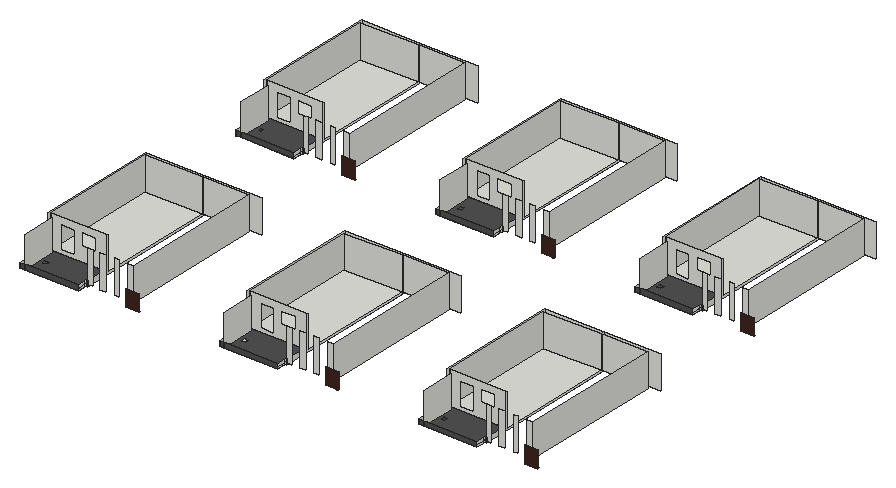
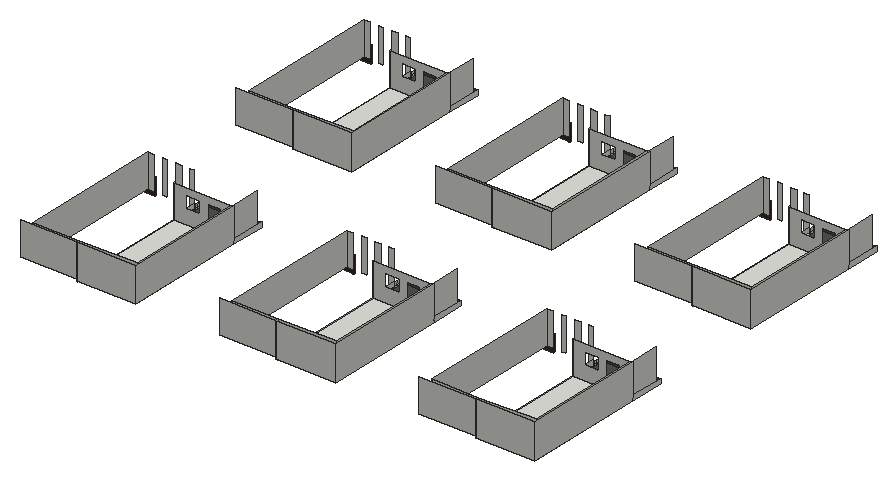
# SketchUp Ruby script. Lengths in inches.
U = 1.inch
M = Sketchup.active_model
def pt(a) = Geom::Point3d.new(a.map { |v| v * U })
def face(e, loops, mat)
  f = e.add_face(loops[0].map { |a| pt(a) })
  loops[1..].each { |l| e.add_face(l.map { |a| pt(a) }).erase! }
  f.material = f.back_material = mat if mat
  f
end
# faces: each face lists its corners as indices into pts; further lists are holes
def faces(e, pts, list, mat = nil) = list.each { |f| face(e, (f[0].is_a?(Array) ? f : [f]).map { |l| l.map { |i| pts[i] } }, mat) }
# xy, xz, yz: faces in a plane at the given z, y or x. An outline is a flat list of corners, or four numbers for a rectangle; further outlines are holes
def ring(l) = l.size == 4 ? [[l[0], l[1]], [l[2], l[1]], [l[2], l[3]], [l[0], l[3]]] : l.each_slice(2).to_a
def flat(e, list, mat, &to3) = list.each { |f| face(e, (f[0].is_a?(Array) ? f : [f]).map { |l| ring(l).map { |u, v| to3.(u, v) } }, mat) }
def xy(e, z, list, mat = nil) = flat(e, list, mat) { |x, y| [x, y, z] }
def xz(e, y, list, mat = nil) = flat(e, list, mat) { |x, z| [x, y, z] }
def yz(e, x, list, mat = nil) = flat(e, list, mat) { |y, z| [x, y, z] }
def lines(e, pts, list) = list.each { |a, b| e.add_line(pt(pts[a]), pt(pts[b])) }
# prism: a flat outline (further loops are holes) pulled along v
def prism(e, loops, v, mat = nil)
  f = face(e, loops, mat); d = Geom::Vector3d.new(v.map { |x| x * U })
  f.pushpull(f.normal.samedirection?(d) ? d.length : -d.length)
end
def box(e, o, s, mat = nil) = prism(e, [[o, [o[0] + s[0], o[1], o[2]], [o[0] + s[0], o[1] + s[1], o[2]], [o[0], o[1] + s[1], o[2]]]], [0, 0, s[2]], mat)
def at(x, y, z, deg = 0) = Geom::Transformation.translation(pt([x, y, z])) * Geom::Transformation.rotation(ORIGIN, Z_AXIS, deg.degrees)
def axes(o, x, y, z) = Geom::Transformation.new([*x, 0, *y, 0, *z, 0, *pt(o).to_a, 1])
def part(name) = M.definitions.add(name)
# library, detail: a bought-in or finely detailed component or shape, given as its bounding box
def library(name, o, s) = part(name).tap { |d| box(d.entities, o, s) }
def detail(e, o, s) = box(e.add_group.entities, o, s)
def put(e, d, t, mat = nil) = e.add_instance(d, t).tap { |i| i.material = mat if mat }
def group(e, t, mat = nil) = e.add_group.tap { |g| g.transformation = t; g.material = mat if mat }.entities
root = M.entities
M.materials.add("[0043_SaddleBrown]").color = [63, 38, 31]
M.materials.add("[0135_DarkGray]").color = [81, 81, 81]
xy(root,114.29,[[500.42,438.72,500.42,441.04,547.05,441.04,547.05,438.73],[1224.86,438.72,1224.86,441.04,1271.49,441.04,1271.49,438.73],[1949.3,438.72,1949.3,441.04,1995.93,441.04,1995.93,438.73],[500.42,1419.07,500.42,1421.39,547.05,1421.39,547.05,1419.08],[1224.86,1419.07,1224.86,1421.39,1271.49,1421.39,1271.49,1419.08],
  [1949.3,1419.07,1949.3,1421.39,1995.93,1421.39,1995.93,1419.08]])
xy(root,126.125,[[348.1875,447.84,353.97,980.35],[1072.625,447.84,1078.41,980.35],[1797.0625,447.84,1802.84,980.35],[891.39,475.13,905.02,487.19],[891.39,567.38,905.02,579.44],
  [891.39,682.44,905.02,694.5],[891.39,858.25,905.02,870.31],[348.1875,1428.19,353.97,1960.7],[1072.625,1428.19,1078.41,1960.7],[1797.0625,1428.19,1802.84,1960.7]])
xy(root,126.125,[[137.5,412.04,153.26,535.375],[[153.26,412.04,348.1875,412.04,348.1875,971.23,137.5,971.23,137.5,535.375,153.26,535.375],[166.95,858.25,180.58,870.31],[166.95,682.44,180.58,694.5],[166.95,567.38,180.58,579.44],[166.95,475.13,180.58,487.19]],[861.9375,412.04,877.69,535.375],[877.69,412.04,877.69,535.375,861.9375,535.375,861.9375,971.23,1072.625,971.23,1072.625,412.04],[1586.375,412.04,1602.13,535.375],
  [[1602.13,412.04,1797.0625,412.04,1797.0625,971.23,1586.375,971.23,1586.375,535.375,1602.13,535.375],[1615.83,858.25,1629.45,870.31],[1615.83,682.44,1629.45,694.5],[1615.83,567.38,1629.45,579.44],[1615.83,475.13,1629.45,487.19]],[166.95,475.13,180.58,487.19],[1615.83,475.13,1629.45,487.19],[166.95,567.38,180.58,579.44],[1615.83,567.38,1629.45,579.44],
  [166.95,682.44,180.58,694.5],[1615.83,682.44,1629.45,694.5],[166.95,858.25,180.58,870.31],[1615.83,858.25,1629.45,870.31],[137.5,1392.39,153.26,1515.73],
  [[153.26,1392.39,348.1875,1392.39,348.1875,1951.58,137.5,1951.58,137.5,1515.73,153.26,1515.73],[166.95,1838.6,180.58,1850.66],[166.95,1662.79,180.58,1674.85],[166.95,1547.73,180.58,1559.79],[166.95,1455.48,180.58,1467.54]],[861.9375,1392.39,877.69,1515.73],[[877.69,1392.39,877.69,1515.73,861.9375,1515.73,861.9375,1951.58,1072.625,1951.58,1072.625,1392.39],[891.39,1455.48,905.02,1467.54],[891.39,1547.73,905.02,1559.79],[891.39,1662.79,905.02,1674.85],[891.39,1838.6,905.02,1850.66]],[1586.375,1392.39,1602.13,1515.73],[[1602.13,1392.39,1797.0625,1392.39,1797.0625,1951.58,1586.375,1951.58,1586.375,1515.73,1602.13,1515.73],[1615.83,1838.6,1629.45,1850.66],[1615.83,1662.79,1629.45,1674.85],[1615.83,1547.73,1629.45,1559.79],[1615.83,1455.48,1629.45,1467.54]],
  [166.95,1455.48,180.58,1467.54],[891.39,1455.48,905.02,1467.54],[1615.83,1455.48,1629.45,1467.54],[166.95,1547.73,180.58,1559.79],[891.39,1547.73,905.02,1559.79],
  [1615.83,1547.73,1629.45,1559.79],[166.95,1662.79,180.58,1674.85],[891.39,1662.79,905.02,1674.85],[1615.83,1662.79,1629.45,1674.85],[166.95,1838.6,180.58,1850.66],
  [891.39,1838.6,905.02,1850.66],[1615.83,1838.6,1629.45,1850.66]],"[0135_DarkGray]")
xy(root,132.25,[[144.84,540.48,353.97,540.48,353.97,971.23,144.84,965.96],[869.28,540.48,1078.41,540.48,1078.41,971.23,869.28,965.96],[1593.72,540.48,1802.84,540.48,1802.84,971.23,1593.72,965.96],[144.84,1520.83,353.97,1520.83,353.97,1951.58,144.84,1946.3125],[869.28,1520.83,1078.41,1520.83,1078.41,1951.58,869.28,1946.3125],
  [1593.72,1520.83,1802.84,1520.83,1802.84,1951.58,1593.72,1946.3125]])
xz(root,412.04,[[137.5,126.125,153.26,143.875],[153.26,126.125,348.1875,143.875],[861.9375,126.125,877.69,143.875],[877.69,126.125,1072.625,143.875],[1586.375,126.125,1602.13,143.875],
  [1602.13,126.125,1797.0625,143.875]],"[0135_DarkGray]")
xz(root,447.84,[[348.1875,126.125,353.97,132.25],[1072.625,126.125,1078.41,132.25],[1797.0625,126.125,1802.84,132.25],[348.1875,132.25,353.97,143.875],[353.97,132.25,370.54,252.25],
  [399.16,132.25,419.76,252.25],[451.01,132.25,467.3,252.25],[500.42,132.25,521.63,252.25],[1072.625,132.25,1078.41,143.875],[1078.41,132.25,1094.98,252.25],
  [1123.6,132.25,1144.2,252.25],[1175.45,132.25,1191.74,252.25],[1224.86,132.25,1246.07,252.25],[1797.0625,132.25,1802.84,143.875],[1802.84,132.25,1819.41,252.25],
  [1848.04,132.25,1868.64,252.25],[1899.89,132.25,1916.17,252.25],[1949.3,132.25,1970.51,252.25]])
xz(root,535.375,[[137.5,126.125,153.26,143.875],[861.9375,126.125,877.69,143.875],[1586.375,126.125,1602.13,143.875]])
xz(root,540.48,[[[144.84,132.25,353.97,252.25],[183.3,143.875,231.3,227.875],[258.09,183.6875,309.84,227.875]],[[869.28,132.25,1078.41,252.25],[907.74,143.875,955.74,227.875],[982.53,183.6875,1034.28,227.875]],[[1593.72,132.25,1802.84,252.25],[1632.17,143.875,1680.17,227.875],[1706.96,183.6875,1758.71,227.875]]])
xz(root,971.23,[[353.97,132.25,521.63,252.25],[1078.41,132.25,1246.07,252.25],[1802.84,132.25,1970.51,252.25]])
xz(root,980.35,[[137.5,126.125,353.97,252.25],[861.9375,126.125,1078.41,252.25],[1586.375,126.125,1802.84,252.25],[353.97,132.25,558.625,252.25],[1078.41,132.25,1283.0625,252.25],
  [1802.84,132.25,2007.5,252.25]])
xz(root,1392.39,[[137.5,126.125,153.26,143.875],[153.26,126.125,348.1875,143.875],[861.9375,126.125,877.69,143.875],[877.69,126.125,1072.625,143.875],[1586.375,126.125,1602.13,143.875],
  [1602.13,126.125,1797.0625,143.875]],"[0135_DarkGray]")
xz(root,1428.19,[[348.1875,126.125,353.97,132.25],[1072.625,126.125,1078.41,132.25],[1797.0625,126.125,1802.84,132.25],[348.1875,132.25,353.97,143.875],[353.97,132.25,370.54,252.25],
  [399.16,132.25,419.76,252.25],[451.01,132.25,467.3,252.25],[500.42,132.25,521.63,252.25],[1072.625,132.25,1078.41,143.875],[1078.41,132.25,1094.98,252.25],
  [1123.6,132.25,1144.2,252.25],[1175.45,132.25,1191.74,252.25],[1224.86,132.25,1246.07,252.25],[1797.0625,132.25,1802.84,143.875],[1802.84,132.25,1819.41,252.25],
  [1848.04,132.25,1868.64,252.25],[1899.89,132.25,1916.17,252.25],[1949.3,132.25,1970.51,252.25]])
xz(root,1515.73,[[137.5,126.125,153.26,143.875],[861.9375,126.125,877.69,143.875],[1586.375,126.125,1602.13,143.875]])
xz(root,1520.83,[[[144.84,132.25,353.97,252.25],[183.3,143.875,231.3,227.875],[258.09,183.6875,309.84,227.875]],[[869.28,132.25,1078.41,252.25],[907.74,143.875,955.74,227.875],[982.53,183.6875,1034.28,227.875]],[[1593.72,132.25,1802.84,252.25],[1632.17,143.875,1680.17,227.875],[1706.96,183.6875,1758.71,227.875]]])
xz(root,1951.58,[[353.97,132.25,521.63,252.25],[1078.41,132.25,1246.07,252.25],[1802.84,132.25,1970.51,252.25]])
xz(root,1960.7,[[137.5,126.125,353.97,252.25],[861.9375,126.125,1078.41,252.25],[1586.375,126.125,1802.84,252.25],[353.97,132.25,558.625,252.25],[1078.41,132.25,1283.0625,252.25],
  [1802.84,132.25,2007.5,252.25]])
yz(root,137.5,[[412.04,126.125,535.375,143.875],[535.375,126.125,980.35,252.25],[1392.39,126.125,1515.73,143.875],[1515.73,126.125,1960.7,252.25]])
yz(root,144.84,[[540.48,132.25,965.96,252.25],[1520.83,132.25,1946.3125,252.25]])
yz(root,153.26,[[412.04,126.125,535.375,240.625],[1392.39,126.125,1515.73,240.625]])
yz(root,348.1875,[[412.04,126.125,438.72,132.25],[438.72,126.125,447.84,132.25],[1392.39,126.125,1419.07,132.25],[1419.07,126.125,1428.19,132.25],[412.04,132.25,438.72,143.875],
  [438.72,132.25,447.84,143.875],[1392.39,132.25,1419.07,143.875],[1419.07,132.25,1428.19,143.875]])
yz(root,353.97,[[447.84,126.125,971.23,126.125,971.23,132.25,540.48,132.25,540.48,252.25,535.375,252.25,535.375,143.875,447.84,143.875],[971.23,126.125,980.35,132.25],[1428.19,126.125,1951.58,126.125,1951.58,132.25,1520.83,132.25,1520.83,252.25,1515.73,252.25,1515.73,143.875,1428.19,143.875],[1951.58,126.125,1960.7,132.25],[971.23,132.25,980.35,252.25],
  [1951.58,132.25,1960.7,252.25]])
yz(root,521.63,[[447.84,132.25,971.23,252.25],[1428.19,132.25,1951.58,252.25]])
yz(root,861.9375,[[412.04,126.125,535.375,143.875],[535.375,126.125,980.35,252.25],[1392.39,126.125,1515.73,143.875],[1515.73,126.125,1960.7,252.25]])
yz(root,869.28,[[540.48,132.25,965.96,252.25],[1520.83,132.25,1946.3125,252.25]])
yz(root,877.69,[[412.04,126.125,535.375,240.625],[1392.39,126.125,1515.73,240.625]])
yz(root,1072.625,[[412.04,126.125,438.72,132.25],[438.72,126.125,447.84,132.25],[1392.39,126.125,1419.07,132.25],[1419.07,126.125,1428.19,132.25],[412.04,132.25,438.72,143.875],
  [438.72,132.25,447.84,143.875],[1392.39,132.25,1419.07,143.875],[1419.07,132.25,1428.19,143.875]])
yz(root,1078.41,[[447.84,126.125,971.23,126.125,971.23,132.25,540.48,132.25,540.48,252.25,535.375,252.25,535.375,143.875,447.84,143.875],[971.23,126.125,980.35,132.25],[1428.19,126.125,1951.58,126.125,1951.58,132.25,1520.83,132.25,1520.83,252.25,1515.73,252.25,1515.73,143.875,1428.19,143.875],[1951.58,126.125,1960.7,132.25],[971.23,132.25,980.35,252.25],
  [1951.58,132.25,1960.7,252.25]])
yz(root,1246.07,[[447.84,132.25,971.23,252.25],[1428.19,132.25,1951.58,252.25]])
yz(root,1586.375,[[412.04,126.125,535.375,143.875],[535.375,126.125,980.35,252.25],[1392.39,126.125,1515.73,143.875],[1515.73,126.125,1960.7,252.25]])
yz(root,1593.72,[[540.48,132.25,965.96,252.25],[1520.83,132.25,1946.3125,252.25]])
yz(root,1602.13,[[412.04,126.125,535.375,240.625],[1392.39,126.125,1515.73,240.625]])
yz(root,1797.0625,[[412.04,126.125,438.72,132.25],[438.72,126.125,447.84,132.25],[1392.39,126.125,1419.07,132.25],[1419.07,126.125,1428.19,132.25],[412.04,132.25,438.72,143.875],
  [438.72,132.25,447.84,143.875],[1392.39,132.25,1419.07,143.875],[1419.07,132.25,1428.19,143.875]])
yz(root,1802.84,[[447.84,126.125,971.23,126.125,971.23,132.25,540.48,132.25,540.48,252.25,535.375,252.25,535.375,143.875,447.84,143.875],[971.23,126.125,980.35,132.25],[1428.19,126.125,1951.58,126.125,1951.58,132.25,1520.83,132.25,1520.83,252.25,1515.73,252.25,1515.73,143.875,1428.19,143.875],[1951.58,126.125,1960.7,132.25],[971.23,132.25,980.35,252.25],
  [1951.58,132.25,1960.7,252.25]])
yz(root,1970.51,[[447.84,132.25,971.23,252.25],[1428.19,132.25,1951.58,252.25]])
p = [[500.42,438.73,174.81],[500.42,438.72,114.29],[547.05,438.73,114.29],[547.05,438.73,174.81],[1224.86,438.73,174.81],[1224.86,438.72,114.29],
  [1271.49,438.73,114.29],[1271.49,438.73,174.81],[1949.3,438.73,174.81],[1949.3,438.72,114.29],[1995.93,438.73,114.29],[1995.93,438.73,174.81],
  [500.42,1419.08,174.81],[500.42,1419.07,114.29],[547.05,1419.08,114.29],[547.05,1419.08,174.81],[1224.86,1419.08,174.81],[1224.86,1419.07,114.29],
  [1271.49,1419.08,114.29],[1271.49,1419.08,174.81],[1949.3,1419.08,174.81],[1949.3,1419.07,114.29],[1995.93,1419.08,114.29],[1995.93,1419.08,174.81],
  [144.84,965.96,132.25],[353.97,971.23,132.25],[353.97,971.23,252.25],[144.84,965.96,252.25],[869.28,965.96,132.25],[1078.41,971.23,132.25],
  [1078.41,971.23,252.25],[869.28,965.96,252.25],[1593.72,965.96,132.25],[1802.84,971.23,132.25],[1802.84,971.23,252.25],[1593.72,965.96,252.25],
  [144.84,1946.3125,132.25],[353.97,1951.58,132.25],[353.97,1951.58,252.25],[144.84,1946.3125,252.25],[869.28,1946.3125,132.25],[1078.41,1951.58,132.25],
  [1078.41,1951.58,252.25],[869.28,1946.3125,252.25],[1593.72,1946.3125,132.25],[1802.84,1951.58,132.25],[1802.84,1951.58,252.25],[1593.72,1946.3125,252.25]]
faces(root,p,[[0,1,2,3],[4,5,6,7],[8,9,10,11],[12,13,14,15],[16,17,18,19],[20,21,22,23]],"[0043_SaddleBrown]")
faces(root,p,[[24,25,26,27],[28,29,30,31],[32,33,34,35],[36,37,38,39],[40,41,42,43],[44,45,46,47]])
